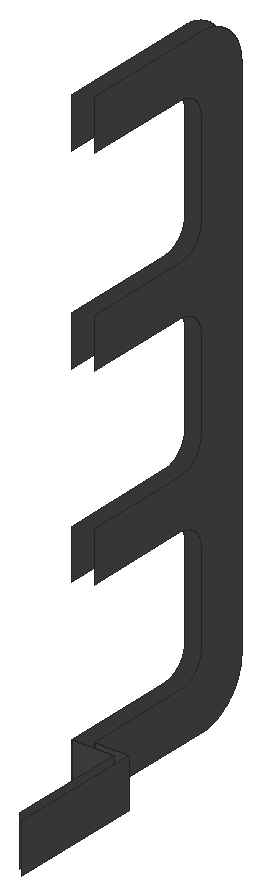
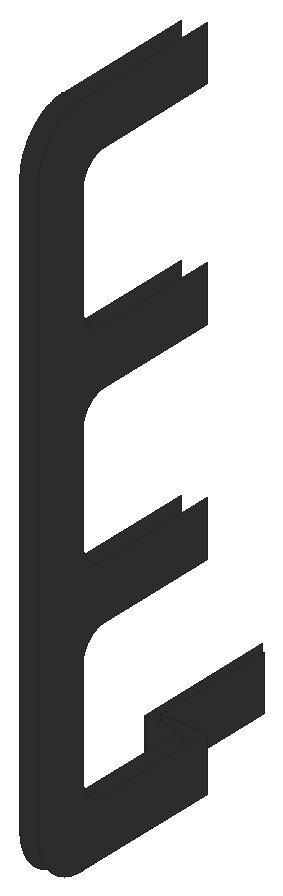
# SketchUp Ruby script. Lengths in inches.
U = 1.inch
M = Sketchup.active_model
def pt(a) = Geom::Point3d.new(a.map { |v| v * U })
def face(e, loops, mat)
  f = e.add_face(loops[0].map { |a| pt(a) })
  loops[1..].each { |l| e.add_face(l.map { |a| pt(a) }).erase! }
  f.material = f.back_material = mat if mat
  f
end
# faces: each face lists its corners as indices into pts; further lists are holes
def faces(e, pts, list, mat = nil) = list.each { |f| face(e, (f[0].is_a?(Array) ? f : [f]).map { |l| l.map { |i| pts[i] } }, mat) }
# xy, xz, yz: faces in a plane at the given z, y or x. An outline is a flat list of corners, or four numbers for a rectangle; further outlines are holes
def ring(l) = l.size == 4 ? [[l[0], l[1]], [l[2], l[1]], [l[2], l[3]], [l[0], l[3]]] : l.each_slice(2).to_a
def flat(e, list, mat, &to3) = list.each { |f| face(e, (f[0].is_a?(Array) ? f : [f]).map { |l| ring(l).map { |u, v| to3.(u, v) } }, mat) }
def xy(e, z, list, mat = nil) = flat(e, list, mat) { |x, y| [x, y, z] }
def xz(e, y, list, mat = nil) = flat(e, list, mat) { |x, z| [x, y, z] }
def yz(e, x, list, mat = nil) = flat(e, list, mat) { |y, z| [x, y, z] }
def lines(e, pts, list) = list.each { |a, b| e.add_line(pt(pts[a]), pt(pts[b])) }
# prism: a flat outline (further loops are holes) pulled along v
def prism(e, loops, v, mat = nil)
  f = face(e, loops, mat); d = Geom::Vector3d.new(v.map { |x| x * U })
  f.pushpull(f.normal.samedirection?(d) ? d.length : -d.length)
end
def box(e, o, s, mat = nil) = prism(e, [[o, [o[0] + s[0], o[1], o[2]], [o[0] + s[0], o[1] + s[1], o[2]], [o[0], o[1] + s[1], o[2]]]], [0, 0, s[2]], mat)
def at(x, y, z, deg = 0) = Geom::Transformation.translation(pt([x, y, z])) * Geom::Transformation.rotation(ORIGIN, Z_AXIS, deg.degrees)
def axes(o, x, y, z) = Geom::Transformation.new([*x, 0, *y, 0, *z, 0, *pt(o).to_a, 1])
def part(name) = M.definitions.add(name)
# library, detail: a bought-in or finely detailed component or shape, given as its bounding box
def library(name, o, s) = part(name).tap { |d| box(d.entities, o, s) }
def detail(e, o, s) = box(e.add_group.entities, o, s)
def put(e, d, t, mat = nil) = e.add_instance(d, t).tap { |i| i.material = mat if mat }
def group(e, t, mat = nil) = e.add_group.tap { |g| g.transformation = t; g.material = mat if mat }.entities
root = M.entities
M.materials.add("1432 AP 8245 TAR ROAD").color = [71, 72, 75]
xy(root,143.79,[[573,431.37,585,431.65]],"1432 AP 8245 TAR ROAD")
xy(root,143.8,[[573,431.94,585,432.22]],"1432 AP 8245 TAR ROAD")
xz(root,329.37,[[573,143.79,603,179.79]],"1432 AP 8245 TAR ROAD")
xz(root,335.37,[[585,143.79,609,179.79]],"1432 AP 8245 TAR ROAD")
yz(root,573,[[329.37,143.79,329.37,179.79,413.61,179.79,413.84,179.8,414.08,179.81,414.3125,179.82,414.55,179.83,414.78,179.85,415.02,179.87,415.25,179.89,415.49,179.92,415.95,179.98,416.1875,180.01,416.42,180.05,416.65,180.09,417.57,180.29,418.26,180.47,418.48,180.53,418.71,180.6,418.93,180.67,419.16,180.75,419.38,180.82,419.6,180.9,419.82,180.99,420.04,181.07,420.48,181.25,420.69,181.35,420.91,181.45,421.54,181.75,421.96,181.97,422.17,182.09,422.37,182.2,422.77,182.44,423.57,182.96,423.76,183.09,424.33,183.51,424.51,183.66,424.7,183.8,425.06,184.1,425.24,184.26,425.41,184.42,425.59,184.57,425.76,184.74,425.93,184.9,426.1,185.0625,426.26,185.23,426.43,185.4,426.59,185.57,426.75,185.75,426.9,185.92,427.06,186.1,427.36,186.46,427.51,186.65,427.65,186.83,428.07,187.4,428.2,187.6,428.34,187.79,428.47,187.99,428.59,188.1875,428.72,188.39,428.96,188.79,429.07,189,429.1875,189.2,429.3,189.41,429.41,189.62,429.51,189.83,429.62,190.04,429.72,190.26,429.8125,190.47,429.91,190.6875,430,190.9,430.09,191.12,430.17,191.34,430.26,191.5625,430.34,191.78,430.41,192.01,430.49,192.23,430.56,192.45,430.63,192.68,430.69,192.91,430.76,193.13,430.82,193.36,430.87,193.59,430.93,193.82,430.98,194.05,431.02,194.28,431.07,194.51,431.11,194.74,431.15,194.98,431.18,195.21,431.22,195.44,431.25,195.68,431.27,195.91,431.29,196.15,431.3125,196.38,431.33,196.61,431.35,196.85,431.36,197.09,431.36,197.32,431.37,197.56,431.37,264.03,431.36,264.26,431.36,264.5,431.35,264.73,431.33,264.97,431.3125,265.2,431.29,265.4375,431.27,265.67,431.25,265.91,431.22,266.14,431.18,266.375,431.15,266.61,431.07,267.07,431.02,267.3,430.98,267.53,430.93,267.76,430.87,267.99,430.82,268.22,430.76,268.45,430.69,268.68,430.63,268.9,430.56,269.13,430.49,269.35,430.41,269.58,430.34,269.8,430.26,270.02,430.17,270.24,430.09,270.46,429.91,270.9,429.8125,271.11,429.72,271.33,429.62,271.54,429.51,271.75,429.41,271.96,429.3,272.17,429.1875,272.38,429.07,272.59,428.96,272.79,428.84,273,428.72,273.2,428.59,273.4,428.47,273.6,428.34,273.79,428.2,273.99,428.07,274.18,427.93,274.37,427.79,274.5625,427.51,274.9375,427.36,275.12,427.06,275.48,426.9,275.66,426.75,275.84,426.43,276.18,426.26,276.35,426.1,276.52,425.93,276.69,425.59,277.01,425.41,277.17,425.24,277.33,424.7,277.78,424.51,277.93,424.33,278.07,423.76,278.49,423.57,278.625,423.37,278.76,422.97,279.02,422.17,279.5,421.54,279.83,421.33,279.9375,421.12,280.04,420.91,280.14,420.69,280.24,420.48,280.33,419.82,280.6,419.16,280.84,418.93,280.91,418.71,280.98,418.48,281.05,418.26,281.12,417.8,281.24,417.57,281.29,417.34,281.35,416.88,281.45,416.42,281.53,416.1875,281.57,415.95,281.61,415.49,281.67,415.25,281.69,415.02,281.72,414.78,281.74,414.55,281.75,414.3125,281.77,414.08,281.78,413.84,281.79,329.37,281.79,329.37,317.79,413.61,317.79,413.84,317.8,414.08,317.81,414.3125,317.82,414.55,317.83,414.78,317.85,415.02,317.87,415.25,317.89,415.49,317.92,415.95,317.98,416.1875,318.01,416.42,318.05,416.65,318.09,417.57,318.29,418.26,318.47,418.48,318.53,418.71,318.6,418.93,318.67,419.16,318.75,419.38,318.82,419.6,318.9,419.82,318.99,420.04,319.07,420.48,319.25,420.69,319.35,420.91,319.45,421.54,319.75,421.96,319.97,422.17,320.09,422.37,320.2,422.77,320.44,423.57,320.96,423.76,321.09,424.33,321.51,424.51,321.66,424.7,321.8,425.06,322.1,425.24,322.26,425.41,322.42,425.59,322.57,425.76,322.74,425.93,322.9,426.1,323.0625,426.26,323.23,426.43,323.4,426.59,323.57,426.75,323.75,426.9,323.92,427.06,324.1,427.36,324.46,427.51,324.65,427.65,324.83,428.07,325.4,428.2,325.6,428.34,325.79,428.47,325.99,428.59,326.1875,428.72,326.39,428.96,326.79,429.07,327,429.1875,327.2,429.3,327.41,429.41,327.62,429.51,327.83,429.62,328.04,429.72,328.26,429.8125,328.47,429.91,328.6875,430,328.9,430.09,329.12,430.17,329.34,430.26,329.5625,430.34,329.78,430.41,330.01,430.49,330.23,430.56,330.45,430.63,330.68,430.69,330.91,430.76,331.13,430.82,331.36,430.87,331.59,430.93,331.82,430.98,332.05,431.02,332.28,431.07,332.51,431.11,332.74,431.15,332.98,431.18,333.21,431.22,333.44,431.25,333.68,431.27,333.91,431.29,334.15,431.3125,334.38,431.33,334.61,431.35,334.85,431.36,335.09,431.36,335.32,431.37,335.56,431.37,402.03,431.36,402.26,431.36,402.5,431.35,402.73,431.33,402.97,431.3125,403.2,431.29,403.4375,431.27,403.67,431.25,403.91,431.22,404.14,431.18,404.375,431.15,404.61,431.07,405.07,431.02,405.3,430.98,405.53,430.93,405.76,430.87,405.99,430.82,406.22,430.76,406.45,430.69,406.68,430.63,406.9,430.56,407.13,430.49,407.35,430.41,407.58,430.34,407.8,430.26,408.02,430.17,408.24,430.09,408.46,429.91,408.9,429.8125,409.11,429.72,409.33,429.62,409.54,429.51,409.75,429.41,409.96,429.3,410.17,429.1875,410.38,429.07,410.59,428.96,410.79,428.84,411,428.72,411.2,428.59,411.4,428.47,411.6,428.34,411.79,428.2,411.99,428.07,412.18,427.93,412.37,427.79,412.5625,427.51,412.9375,427.36,413.12,427.06,413.48,426.9,413.66,426.75,413.84,426.43,414.18,426.26,414.35,426.1,414.52,425.93,414.69,425.59,415.01,425.41,415.17,425.24,415.33,424.7,415.78,424.51,415.93,424.33,416.07,423.76,416.49,423.57,416.625,423.37,416.76,422.97,417.02,422.17,417.5,421.54,417.83,421.33,417.9375,421.12,418.04,420.91,418.14,420.69,418.24,420.48,418.33,419.82,418.6,419.16,418.84,418.93,418.91,418.71,418.98,418.48,419.05,418.26,419.12,417.8,419.24,417.57,419.29,417.34,419.35,416.88,419.45,416.42,419.53,416.1875,419.57,415.95,419.61,415.49,419.67,415.25,419.69,415.02,419.72,414.78,419.74,414.55,419.75,414.3125,419.77,414.08,419.78,413.84,419.79,329.37,419.79,329.37,455.79,413.61,455.79,413.84,455.8,414.08,455.81,414.3125,455.82,414.55,455.83,414.78,455.85,415.02,455.87,415.25,455.89,415.49,455.92,415.95,455.98,416.1875,456.01,416.42,456.05,416.65,456.09,417.57,456.29,418.26,456.47,418.48,456.53,418.71,456.6,418.93,456.67,419.16,456.75,419.38,456.82,419.6,456.9,419.82,456.99,420.04,457.07,420.48,457.25,420.69,457.35,420.91,457.45,421.54,457.75,421.96,457.97,422.17,458.09,422.37,458.2,422.77,458.44,423.57,458.96,423.76,459.09,424.33,459.51,424.51,459.66,424.7,459.8,425.06,460.1,425.24,460.26,425.41,460.42,425.59,460.57,425.76,460.74,425.93,460.9,426.1,461.0625,426.26,461.23,426.43,461.4,426.59,461.57,426.75,461.75,426.9,461.92,427.06,462.1,427.36,462.46,427.51,462.65,427.65,462.83,428.07,463.4,428.2,463.6,428.34,463.79,428.47,463.99,428.59,464.1875,428.72,464.39,428.96,464.79,429.07,465,429.1875,465.2,429.3,465.41,429.41,465.62,429.51,465.83,429.62,466.04,429.72,466.26,429.8125,466.47,429.91,466.6875,430,466.9,430.09,467.12,430.17,467.34,430.26,467.5625,430.34,467.78,430.41,468.01,430.49,468.23,430.56,468.45,430.63,468.68,430.69,468.91,430.76,469.13,430.82,469.36,430.87,469.59,430.93,469.82,430.98,470.05,431.02,470.28,431.07,470.51,431.11,470.74,431.15,470.98,431.18,471.21,431.22,471.44,431.25,471.68,431.27,471.91,431.29,472.15,431.3125,472.38,431.33,472.61,431.35,472.85,431.36,473.09,431.36,473.32,431.37,473.56,431.37,543.03,431.36,543.26,431.36,543.5,431.35,543.73,431.33,543.97,431.3125,544.2,431.29,544.4375,431.27,544.67,431.25,544.91,431.22,545.14,431.18,545.375,431.15,545.61,431.07,546.07,431.02,546.3,430.98,546.53,430.93,546.76,430.87,546.99,430.82,547.22,430.76,547.45,430.69,547.68,430.63,547.9,430.56,548.13,430.49,548.35,430.41,548.58,430.34,548.8,430.26,549.02,430.17,549.24,430.09,549.46,429.91,549.9,429.8125,550.11,429.72,550.33,429.62,550.54,429.51,550.75,429.41,550.96,429.3,551.17,429.1875,551.38,429.07,551.59,428.96,551.79,428.84,552,428.72,552.2,428.59,552.4,428.47,552.6,428.34,552.79,428.2,552.99,428.07,553.18,427.93,553.37,427.79,553.5625,427.51,553.9375,427.36,554.12,427.06,554.48,426.9,554.66,426.75,554.84,426.43,555.18,426.26,555.35,426.1,555.52,425.93,555.69,425.59,556.01,425.41,556.17,425.24,556.33,424.7,556.78,424.51,556.93,424.33,557.07,423.76,557.49,423.57,557.625,423.37,557.76,422.97,558.02,422.17,558.5,421.54,558.83,421.33,558.9375,421.12,559.04,420.91,559.14,420.69,559.24,420.48,559.33,419.82,559.6,419.16,559.84,418.93,559.91,418.71,559.98,418.48,560.05,418.26,560.12,417.8,560.24,417.57,560.29,417.34,560.35,416.88,560.45,416.42,560.53,416.1875,560.57,415.95,560.61,415.49,560.67,415.25,560.69,415.02,560.72,414.78,560.74,414.55,560.75,414.3125,560.77,414.08,560.78,413.84,560.79,329.37,560.79,329.37,596.79,431.94,596.79,432.78,596.76,433.07,596.75,433.35,596.74,434.19,596.68,434.48,596.66,435.88,596.51,437,596.35,437.28,596.3,437.56,596.26,437.84,596.21,438.12,596.15,438.39,596.1,438.67,596.04,438.95,595.99,439.22,595.93,439.5,595.86,439.77,595.8,440.05,595.73,440.32,595.66,440.6,595.59,440.87,595.52,441.68,595.28,441.96,595.2,442.23,595.12,442.49,595.03,443.3,594.76,443.5625,594.66,443.83,594.57,444.1,594.47,444.36,594.37,444.62,594.26,444.88,594.16,445.15,594.05,445.93,593.72,446.18,593.6,446.44,593.49,446.7,593.37,446.95,593.24,447.21,593.12,447.46,593,447.71,592.87,447.97,592.74,448.22,592.61,448.46,592.47,448.71,592.34,448.96,592.2,449.21,592.0625,449.45,591.92,449.7,591.78,449.9375,591.63,450.18,591.49,450.42,591.34,450.66,591.1875,450.9,591.04,451.13,590.88,451.37,590.72,451.6,590.57,451.84,590.41,452.07,590.25,452.3,590.08,452.53,589.92,452.99,589.58,453.43,589.24,453.66,589.0625,453.88,588.89,454.32,588.53,454.53,588.35,454.75,588.17,454.96,587.98,455.18,587.8,455.81,587.23,456.01,587.03,456.22,586.84,456.42,586.64,456.625,586.45,456.83,586.25,457.02,586.05,457.22,585.84,457.42,585.64,457.61,585.4375,457.81,585.23,458,585.02,458.1875,584.8125,458.375,584.6,458.56,584.39,458.74,584.17,458.93,583.96,459.47,583.3,459.64,583.08,459.82,582.86,459.99,582.63,460.16,582.41,460.33,582.18,460.49,581.95,460.66,581.72,461.14,581.03,461.3,580.79,461.46,580.56,461.61,580.32,461.77,580.08,461.92,579.84,462.06,579.6,462.36,579.12,462.64,578.63,462.78,578.38,462.92,578.14,463.05,577.89,463.19,577.64,463.45,577.14,463.57,576.88,463.7,576.63,463.94,576.12,464.0625,575.86,464.18,575.61,464.3,575.35,464.74,574.31,464.84,574.04,464.94,573.78,465.05,573.52,465.14,573.25,465.24,572.99,465.34,572.72,465.43,572.45,465.52,572.19,465.61,571.92,465.69,571.65,465.78,571.38,465.94,570.84,466.02,570.5625,466.09,570.29,466.17,570.02,466.24,569.74,466.31,569.47,466.375,569.2,466.44,568.92,466.5,568.65,466.5625,568.37,466.62,568.09,466.68,567.82,466.93,566.42,467.09,565.3,467.24,563.9,467.26,563.62,467.28,563.33,467.32,562.77,467.34,562.21,467.35,561.92,467.37,561.36,467.37,179.23,467.36,178.94,467.33,178.1,467.32,177.8125,467.3,177.53,467.26,176.97,467.24,176.6875,467.21,176.4,467.15,175.84,467.12,175.5625,467.09,175.28,466.93,174.16,466.78,173.32,466.73,173.05,466.68,172.77,466.62,172.49,466.5625,172.22,466.5,171.9375,466.44,171.66,466.375,171.39,466.31,171.11,466.17,170.57,466.09,170.29,466.02,170.02,465.78,169.21,465.69,168.9375,465.61,168.67,465.34,167.86,465.24,167.6,465.14,167.33,465.05,167.07,464.94,166.8,464.74,166.28,464.63,166.02,464.52,165.75,464.41,165.49,464.3,165.24,464.18,164.98,464.0625,164.72,463.94,164.46,463.82,164.21,463.7,163.95,463.57,163.7,463.45,163.45,463.19,162.95,463.05,162.7,462.92,162.45,462.78,162.2,462.64,161.96,462.5,161.71,462.36,161.47,462.21,161.22,462.06,160.98,461.92,160.74,461.77,160.5,461.61,160.26,461.46,160.03,461.3,159.79,461.14,159.56,460.98,159.32,460.66,158.86,460.49,158.63,460.33,158.4,460.16,158.18,459.99,157.95,459.82,157.73,459.64,157.5,459.47,157.28,459.29,157.0625,459.11,156.84,458.93,156.63,458.74,156.41,458.56,156.2,458.375,155.98,458.1875,155.77,458,155.5625,457.81,155.36,457.61,155.15,457.42,154.94,457.02,154.54,456.83,154.34,456.42,153.94,456.22,153.74,456.01,153.55,455.81,153.36,455.18,152.79,454.96,152.6,454.75,152.42,454.53,152.23,454.32,152.05,453.88,151.7,453.66,151.52,453.43,151.35,453.21,151.17,452.99,151,452.76,150.83,452.53,150.67,452.3,150.5,451.84,150.18,451.6,150.02,451.37,149.86,451.13,149.7,450.9,149.55,450.18,149.1,449.9375,148.95,449.7,148.81,449.45,148.66,449.21,148.52,448.96,148.38,448.71,148.25,448.46,148.11,448.22,147.98,447.97,147.85,447.71,147.72,447.21,147.46,446.95,147.34,446.7,147.22,446.18,146.98,445.93,146.87,445.67,146.75,445.15,146.53,444.88,146.43,444.62,146.32,444.1,146.12,443.83,146.02,443.5625,145.92,443.3,145.83,443.03,145.73,442.49,145.55,442.23,145.47,441.96,145.38,441.68,145.3,441.14,145.14,440.87,145.07,440.6,144.99,440.32,144.92,440.05,144.85,439.77,144.79,439.5,144.72,439.22,144.66,438.95,144.6,438.39,144.48,438.12,144.43,437.28,144.28,437,144.24,436.72,144.19,436.16,144.11,435.88,144.08,435.6,144.04,434.76,143.95,434.48,143.93,434.19,143.9,433.63,143.86,433.35,143.85,433.07,143.83,432.78,143.82,432.22,143.8,431.94,143.8,431.65,143.79]],"1432 AP 8245 TAR ROAD")
yz(root,585,[[335.37,143.79,431.65,143.79,431.94,143.8,432.22,143.8,432.78,143.82,433.07,143.83,433.35,143.85,433.63,143.86,434.19,143.9,434.48,143.93,434.76,143.95,435.6,144.04,435.88,144.08,436.16,144.11,436.72,144.19,437,144.24,437.28,144.28,438.12,144.43,438.39,144.48,438.95,144.6,439.22,144.66,439.5,144.72,439.77,144.79,440.05,144.85,440.32,144.92,440.6,144.99,440.87,145.07,441.14,145.14,441.68,145.3,441.96,145.38,442.23,145.47,442.49,145.55,443.03,145.73,443.3,145.83,443.5625,145.92,443.83,146.02,444.1,146.12,444.62,146.32,444.88,146.43,445.15,146.53,445.67,146.75,445.93,146.87,446.18,146.98,446.7,147.22,446.95,147.34,447.21,147.46,447.71,147.72,447.97,147.85,448.22,147.98,448.46,148.11,448.71,148.25,448.96,148.38,449.21,148.52,449.45,148.66,449.7,148.81,449.9375,148.95,450.18,149.1,450.9,149.55,451.13,149.7,451.37,149.86,451.6,150.02,451.84,150.18,452.3,150.5,452.53,150.67,452.76,150.83,452.99,151,453.21,151.17,453.43,151.35,453.66,151.52,453.88,151.7,454.32,152.05,454.53,152.23,454.75,152.42,454.96,152.6,455.18,152.79,455.81,153.36,456.01,153.55,456.22,153.74,456.42,153.94,456.83,154.34,457.02,154.54,457.42,154.94,457.61,155.15,457.81,155.36,458,155.5625,458.1875,155.77,458.375,155.98,458.56,156.2,458.74,156.41,458.93,156.63,459.11,156.84,459.29,157.0625,459.47,157.28,459.64,157.5,459.82,157.73,459.99,157.95,460.16,158.18,460.33,158.4,460.49,158.63,460.66,158.86,460.98,159.32,461.14,159.56,461.3,159.79,461.46,160.03,461.61,160.26,461.77,160.5,461.92,160.74,462.06,160.98,462.21,161.22,462.36,161.47,462.5,161.71,462.64,161.96,462.78,162.2,462.92,162.45,463.05,162.7,463.19,162.95,463.45,163.45,463.57,163.7,463.7,163.95,463.82,164.21,463.94,164.46,464.0625,164.72,464.18,164.98,464.3,165.24,464.41,165.49,464.52,165.75,464.63,166.02,464.74,166.28,464.94,166.8,465.05,167.07,465.14,167.33,465.24,167.6,465.34,167.86,465.61,168.67,465.69,168.9375,465.78,169.21,466.02,170.02,466.09,170.29,466.17,170.57,466.31,171.11,466.375,171.39,466.44,171.66,466.5,171.9375,466.5625,172.22,466.62,172.49,466.68,172.77,466.73,173.05,466.78,173.32,466.93,174.16,467.09,175.28,467.12,175.5625,467.15,175.84,467.21,176.4,467.24,176.6875,467.26,176.97,467.3,177.53,467.32,177.8125,467.33,178.1,467.36,178.94,467.37,179.23,467.37,561.36,467.35,561.92,467.34,562.21,467.32,562.77,467.28,563.33,467.26,563.62,467.24,563.9,467.09,565.3,466.93,566.42,466.68,567.82,466.62,568.09,466.5625,568.37,466.5,568.65,466.44,568.92,466.375,569.2,466.31,569.47,466.24,569.74,466.17,570.02,466.09,570.29,466.02,570.5625,465.94,570.84,465.78,571.38,465.69,571.65,465.61,571.92,465.52,572.19,465.43,572.45,465.34,572.72,465.24,572.99,465.14,573.25,465.05,573.52,464.94,573.78,464.84,574.04,464.74,574.31,464.3,575.35,464.18,575.61,464.0625,575.86,463.94,576.12,463.7,576.63,463.57,576.88,463.45,577.14,463.19,577.64,463.05,577.89,462.92,578.14,462.78,578.38,462.64,578.63,462.36,579.12,462.06,579.6,461.92,579.84,461.77,580.08,461.61,580.32,461.46,580.56,461.3,580.79,461.14,581.03,460.66,581.72,460.49,581.95,460.33,582.18,460.16,582.41,459.99,582.63,459.82,582.86,459.64,583.08,459.47,583.3,458.93,583.96,458.74,584.17,458.56,584.39,458.375,584.6,458.1875,584.8125,458,585.02,457.81,585.23,457.61,585.4375,457.42,585.64,457.22,585.84,457.02,586.05,456.83,586.25,456.625,586.45,456.42,586.64,456.22,586.84,456.01,587.03,455.81,587.23,455.18,587.8,454.96,587.98,454.75,588.17,454.53,588.35,454.32,588.53,453.88,588.89,453.66,589.0625,453.43,589.24,452.99,589.58,452.53,589.92,452.3,590.08,452.07,590.25,451.84,590.41,451.6,590.57,451.37,590.72,451.13,590.88,450.9,591.04,450.66,591.1875,450.42,591.34,450.18,591.49,449.9375,591.63,449.7,591.78,449.45,591.92,449.21,592.0625,448.96,592.2,448.71,592.34,448.46,592.47,448.22,592.61,447.97,592.74,447.71,592.87,447.46,593,447.21,593.12,446.95,593.24,446.7,593.37,446.44,593.49,446.18,593.6,445.93,593.72,445.15,594.05,444.88,594.16,444.62,594.26,444.36,594.37,444.1,594.47,443.83,594.57,443.5625,594.66,443.3,594.76,442.49,595.03,442.23,595.12,441.96,595.2,441.68,595.28,440.87,595.52,440.6,595.59,440.32,595.66,440.05,595.73,439.77,595.8,439.5,595.86,439.22,595.93,438.95,595.99,438.67,596.04,438.39,596.1,438.12,596.15,437.84,596.21,437.56,596.26,437.28,596.3,437,596.35,435.88,596.51,434.48,596.66,434.19,596.68,433.35,596.74,433.07,596.75,432.78,596.76,431.94,596.79,335.37,596.79,335.37,560.79,413.84,560.79,414.08,560.78,414.3125,560.77,414.55,560.75,414.78,560.74,415.02,560.72,415.25,560.69,415.49,560.67,415.95,560.61,416.1875,560.57,416.42,560.53,416.88,560.45,417.34,560.35,417.57,560.29,417.8,560.24,418.26,560.12,418.48,560.05,418.71,559.98,418.93,559.91,419.16,559.84,419.82,559.6,420.48,559.33,420.69,559.24,420.91,559.14,421.12,559.04,421.33,558.9375,421.54,558.83,422.17,558.5,422.97,558.02,423.37,557.76,423.57,557.625,423.76,557.49,424.33,557.07,424.51,556.93,424.7,556.78,425.24,556.33,425.41,556.17,425.59,556.01,425.93,555.69,426.1,555.52,426.26,555.35,426.43,555.18,426.75,554.84,426.9,554.66,427.06,554.48,427.36,554.12,427.51,553.9375,427.79,553.5625,427.93,553.37,428.07,553.18,428.2,552.99,428.34,552.79,428.47,552.6,428.59,552.4,428.72,552.2,428.84,552,428.96,551.79,429.07,551.59,429.1875,551.38,429.3,551.17,429.41,550.96,429.51,550.75,429.62,550.54,429.72,550.33,429.8125,550.11,429.91,549.9,430.09,549.46,430.17,549.24,430.26,549.02,430.34,548.8,430.41,548.58,430.49,548.35,430.56,548.13,430.63,547.9,430.69,547.68,430.76,547.45,430.82,547.22,430.87,546.99,430.93,546.76,430.98,546.53,431.02,546.3,431.07,546.07,431.15,545.61,431.18,545.375,431.22,545.14,431.25,544.91,431.27,544.67,431.29,544.4375,431.3125,544.2,431.33,543.97,431.35,543.73,431.36,543.5,431.36,543.26,431.37,543.03,431.37,473.56,431.36,473.32,431.36,473.09,431.35,472.85,431.33,472.61,431.3125,472.38,431.29,472.15,431.27,471.91,431.25,471.68,431.22,471.44,431.18,471.21,431.15,470.98,431.11,470.74,431.07,470.51,431.02,470.28,430.98,470.05,430.93,469.82,430.87,469.59,430.82,469.36,430.76,469.13,430.69,468.91,430.63,468.68,430.56,468.45,430.49,468.23,430.41,468.01,430.34,467.78,430.26,467.5625,430.17,467.34,430.09,467.12,430,466.9,429.91,466.6875,429.8125,466.47,429.72,466.26,429.62,466.04,429.51,465.83,429.41,465.62,429.3,465.41,429.1875,465.2,429.07,465,428.96,464.79,428.72,464.39,428.59,464.1875,428.47,463.99,428.34,463.79,428.2,463.6,428.07,463.4,427.65,462.83,427.51,462.65,427.36,462.46,427.06,462.1,426.9,461.92,426.75,461.75,426.59,461.57,426.43,461.4,426.26,461.23,426.1,461.0625,425.93,460.9,425.76,460.74,425.59,460.57,425.41,460.42,425.24,460.26,425.06,460.1,424.7,459.8,424.51,459.66,424.33,459.51,423.76,459.09,423.57,458.96,422.77,458.44,422.37,458.2,422.17,458.09,421.96,457.97,421.54,457.75,420.91,457.45,420.69,457.35,420.48,457.25,420.04,457.07,419.82,456.99,419.6,456.9,419.38,456.82,419.16,456.75,418.93,456.67,418.71,456.6,418.48,456.53,418.26,456.47,417.57,456.29,416.65,456.09,416.42,456.05,416.1875,456.01,415.95,455.98,415.49,455.92,415.25,455.89,415.02,455.87,414.78,455.85,414.55,455.83,414.3125,455.82,414.08,455.81,413.84,455.8,413.61,455.79,335.37,455.79,335.37,419.79,413.84,419.79,414.08,419.78,414.3125,419.77,414.55,419.75,414.78,419.74,415.02,419.72,415.25,419.69,415.49,419.67,415.95,419.61,416.1875,419.57,416.42,419.53,416.88,419.45,417.34,419.35,417.57,419.29,417.8,419.24,418.26,419.12,418.48,419.05,418.71,418.98,418.93,418.91,419.16,418.84,419.82,418.6,420.48,418.33,420.69,418.24,420.91,418.14,421.12,418.04,421.33,417.9375,421.54,417.83,422.17,417.5,422.97,417.02,423.37,416.76,423.57,416.625,423.76,416.49,424.33,416.07,424.51,415.93,424.7,415.78,425.24,415.33,425.41,415.17,425.59,415.01,425.93,414.69,426.1,414.52,426.26,414.35,426.43,414.18,426.75,413.84,426.9,413.66,427.06,413.48,427.36,413.12,427.51,412.9375,427.79,412.5625,427.93,412.37,428.07,412.18,428.2,411.99,428.34,411.79,428.47,411.6,428.59,411.4,428.72,411.2,428.84,411,428.96,410.79,429.07,410.59,429.1875,410.38,429.3,410.17,429.41,409.96,429.51,409.75,429.62,409.54,429.72,409.33,429.8125,409.11,429.91,408.9,430.09,408.46,430.17,408.24,430.26,408.02,430.34,407.8,430.41,407.58,430.49,407.35,430.56,407.13,430.63,406.9,430.69,406.68,430.76,406.45,430.82,406.22,430.87,405.99,430.93,405.76,430.98,405.53,431.02,405.3,431.07,405.07,431.15,404.61,431.18,404.375,431.22,404.14,431.25,403.91,431.27,403.67,431.29,403.4375,431.3125,403.2,431.33,402.97,431.35,402.73,431.36,402.5,431.36,402.26,431.37,402.03,431.37,335.56,431.36,335.32,431.36,335.09,431.35,334.85,431.33,334.61,431.3125,334.38,431.29,334.15,431.27,333.91,431.25,333.68,431.22,333.44,431.18,333.21,431.15,332.98,431.11,332.74,431.07,332.51,431.02,332.28,430.98,332.05,430.93,331.82,430.87,331.59,430.82,331.36,430.76,331.13,430.69,330.91,430.63,330.68,430.56,330.45,430.49,330.23,430.41,330.01,430.34,329.78,430.26,329.5625,430.17,329.34,430.09,329.12,430,328.9,429.91,328.6875,429.8125,328.47,429.72,328.26,429.62,328.04,429.51,327.83,429.41,327.62,429.3,327.41,429.1875,327.2,429.07,327,428.96,326.79,428.72,326.39,428.59,326.1875,428.47,325.99,428.34,325.79,428.2,325.6,428.07,325.4,427.65,324.83,427.51,324.65,427.36,324.46,427.06,324.1,426.9,323.92,426.75,323.75,426.59,323.57,426.43,323.4,426.26,323.23,426.1,323.0625,425.93,322.9,425.76,322.74,425.59,322.57,425.41,322.42,425.24,322.26,425.06,322.1,424.7,321.8,424.51,321.66,424.33,321.51,423.76,321.09,423.57,320.96,422.77,320.44,422.37,320.2,422.17,320.09,421.96,319.97,421.54,319.75,420.91,319.45,420.69,319.35,420.48,319.25,420.04,319.07,419.82,318.99,419.6,318.9,419.38,318.82,419.16,318.75,418.93,318.67,418.71,318.6,418.48,318.53,418.26,318.47,417.57,318.29,416.65,318.09,416.42,318.05,416.1875,318.01,415.95,317.98,415.49,317.92,415.25,317.89,415.02,317.87,414.78,317.85,414.55,317.83,414.3125,317.82,414.08,317.81,413.84,317.8,413.61,317.79,335.37,317.79,335.37,281.79,413.84,281.79,414.08,281.78,414.3125,281.77,414.55,281.75,414.78,281.74,415.02,281.72,415.25,281.69,415.49,281.67,415.95,281.61,416.1875,281.57,416.42,281.53,416.88,281.45,417.34,281.35,417.57,281.29,417.8,281.24,418.26,281.12,418.48,281.05,418.71,280.98,418.93,280.91,419.16,280.84,419.82,280.6,420.48,280.33,420.69,280.24,420.91,280.14,421.12,280.04,421.33,279.9375,421.54,279.83,422.17,279.5,422.97,279.02,423.37,278.76,423.57,278.625,423.76,278.49,424.33,278.07,424.51,277.93,424.7,277.78,425.24,277.33,425.41,277.17,425.59,277.01,425.93,276.69,426.1,276.52,426.26,276.35,426.43,276.18,426.75,275.84,426.9,275.66,427.06,275.48,427.36,275.12,427.51,274.9375,427.79,274.5625,427.93,274.37,428.07,274.18,428.2,273.99,428.34,273.79,428.47,273.6,428.59,273.4,428.72,273.2,428.84,273,428.96,272.79,429.07,272.59,429.1875,272.38,429.3,272.17,429.41,271.96,429.51,271.75,429.62,271.54,429.72,271.33,429.8125,271.11,429.91,270.9,430.09,270.46,430.17,270.24,430.26,270.02,430.34,269.8,430.41,269.58,430.49,269.35,430.56,269.13,430.63,268.9,430.69,268.68,430.76,268.45,430.82,268.22,430.87,267.99,430.93,267.76,430.98,267.53,431.02,267.3,431.07,267.07,431.15,266.61,431.18,266.375,431.22,266.14,431.25,265.91,431.27,265.67,431.29,265.4375,431.3125,265.2,431.33,264.97,431.35,264.73,431.36,264.5,431.36,264.26,431.37,264.03,431.37,197.56,431.36,197.32,431.36,197.09,431.35,196.85,431.33,196.61,431.3125,196.38,431.29,196.15,431.27,195.91,431.25,195.68,431.22,195.44,431.18,195.21,431.15,194.98,431.11,194.74,431.07,194.51,431.02,194.28,430.98,194.05,430.93,193.82,430.87,193.59,430.82,193.36,430.76,193.13,430.69,192.91,430.63,192.68,430.56,192.45,430.49,192.23,430.41,192.01,430.34,191.78,430.26,191.5625,430.17,191.34,430.09,191.12,430,190.9,429.91,190.6875,429.8125,190.47,429.72,190.26,429.62,190.04,429.51,189.83,429.41,189.62,429.3,189.41,429.1875,189.2,429.07,189,428.96,188.79,428.72,188.39,428.59,188.1875,428.47,187.99,428.34,187.79,428.2,187.6,428.07,187.4,427.65,186.83,427.51,186.65,427.36,186.46,427.06,186.1,426.9,185.92,426.75,185.75,426.59,185.57,426.43,185.4,426.26,185.23,426.1,185.0625,425.93,184.9,425.76,184.74,425.59,184.57,425.41,184.42,425.24,184.26,425.06,184.1,424.7,183.8,424.51,183.66,424.33,183.51,423.76,183.09,423.57,182.96,422.77,182.44,422.37,182.2,422.17,182.09,421.96,181.97,421.54,181.75,420.91,181.45,420.69,181.35,420.48,181.25,420.04,181.07,419.82,180.99,419.6,180.9,419.38,180.82,419.16,180.75,418.93,180.67,418.71,180.6,418.48,180.53,418.26,180.47,417.57,180.29,416.65,180.09,416.42,180.05,416.1875,180.01,415.95,179.98,415.49,179.92,415.25,179.89,415.02,179.87,414.78,179.85,414.55,179.83,414.3125,179.82,414.08,179.81,413.84,179.8,413.61,179.79,335.37,179.79]],"1432 AP 8245 TAR ROAD")
yz(root,603,[[245.37,143.79,329.37,179.79]],"1432 AP 8245 TAR ROAD")
yz(root,609,[[239.37,143.79,335.37,179.79]],"1432 AP 8245 TAR ROAD")
p = [[573,431.65,143.79],[573,431.94,143.8],[585,431.94,143.8],[585,431.65,143.79],[573,432.22,143.8],[573,432.5,143.81],
  [585,432.5,143.81],[585,432.22,143.8],[573,432.78,143.82],[585,432.78,143.82],[573,433.07,143.83],[585,433.07,143.83],
  [573,433.35,143.85],[585,433.35,143.85],[573,433.63,143.86],[585,433.63,143.86],[573,433.91,143.88],[585,433.91,143.88],
  [573,434.19,143.9],[585,434.19,143.9],[573,434.48,143.93],[585,434.48,143.93]]
faces(root,p,[[0,1,2,3],[4,5,6,7],[5,8,9,6],[8,10,11,9],[10,12,13,11],[12,14,15,13],[14,16,17,15],[16,18,19,17],
  [18,20,21,19]],"1432 AP 8245 TAR ROAD")
